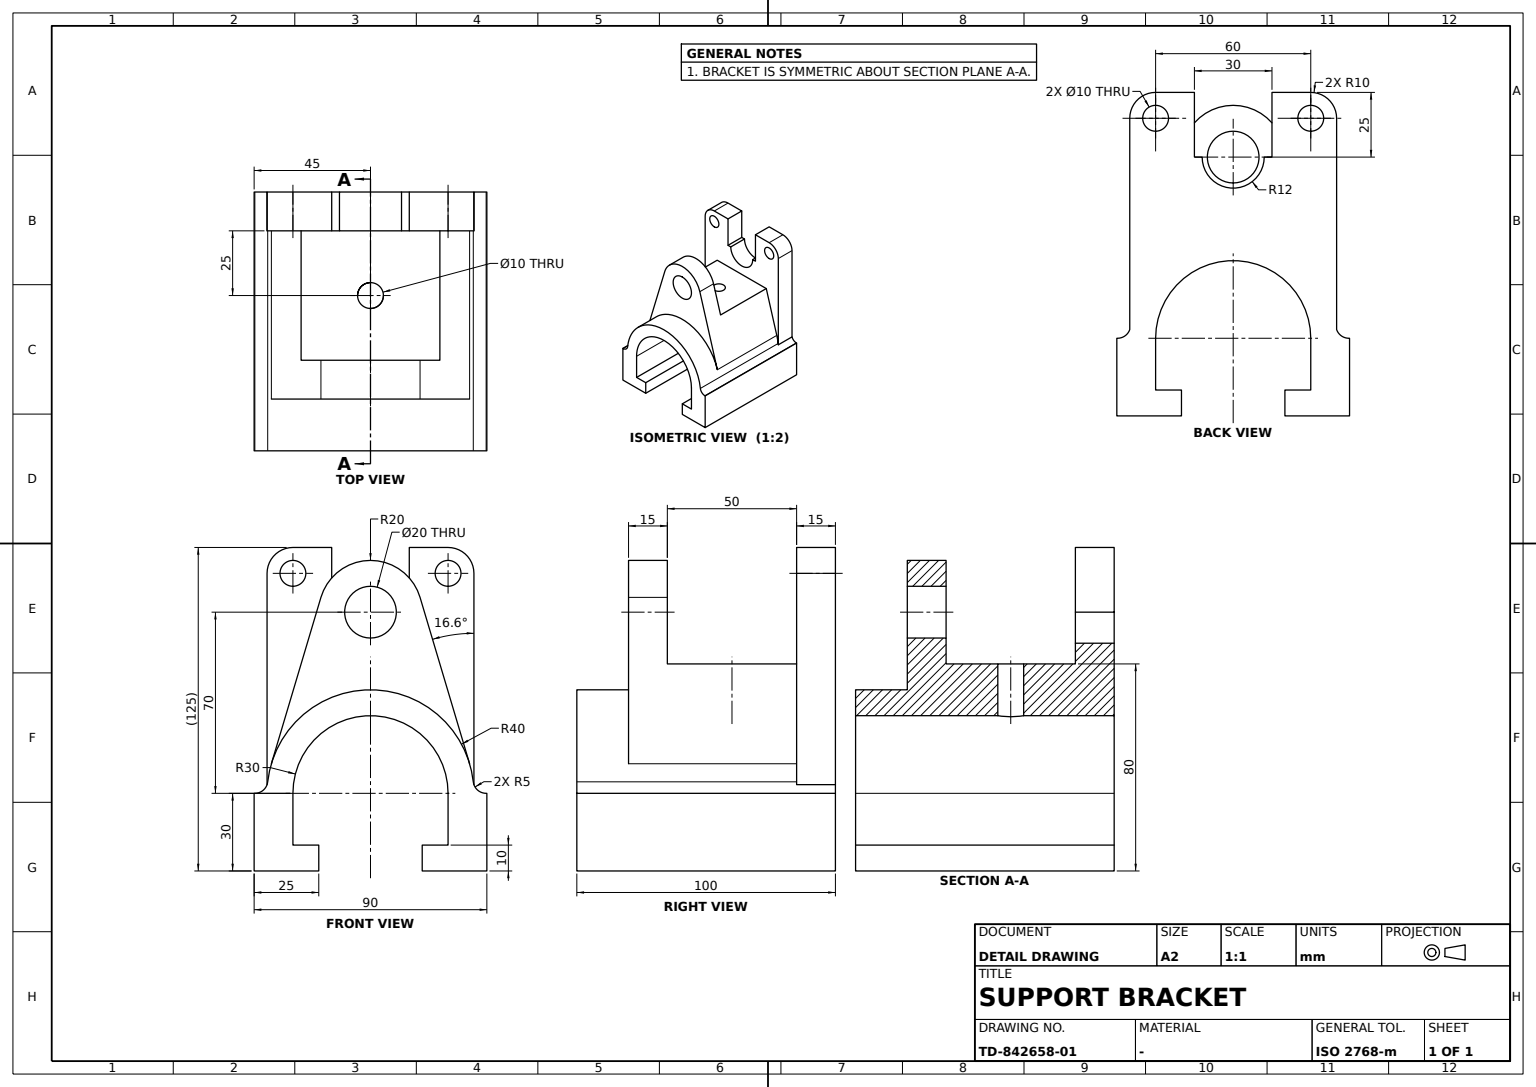
ISO-10303-21;
HEADER;
FILE_DESCRIPTION((''),'2;1');
FILE_NAME('','',(''),(''),'','','');
FILE_SCHEMA(('AUTOMOTIVE_DESIGN'));
ENDSEC;
DATA;
#1=APPLICATION_CONTEXT('');
#2=PRODUCT_CONTEXT('',#1,'mechanical');
#3=PRODUCT('','','',(#2));
#4=PRODUCT_DEFINITION_FORMATION('','',#3);
#5=PRODUCT_DEFINITION_CONTEXT('',#1,'design');
#6=PRODUCT_DEFINITION('','',#4,#5);
#7=PRODUCT_DEFINITION_SHAPE('','',#6);
#8=(LENGTH_UNIT()NAMED_UNIT(*)SI_UNIT(.MILLI.,.METRE.));
#9=(NAMED_UNIT(*)PLANE_ANGLE_UNIT()SI_UNIT($,.RADIAN.));
#10=(NAMED_UNIT(*)SI_UNIT($,.STERADIAN.)SOLID_ANGLE_UNIT());
#11=UNCERTAINTY_MEASURE_WITH_UNIT(LENGTH_MEASURE(0.005),#8,'distance_accuracy_value','');
#12=(GEOMETRIC_REPRESENTATION_CONTEXT(3)GLOBAL_UNCERTAINTY_ASSIGNED_CONTEXT((#11))GLOBAL_UNIT_ASSIGNED_CONTEXT((#8,#9,#10))REPRESENTATION_CONTEXT('',''));
#13=CARTESIAN_POINT('',(38.332594,-35.,41.428571));
#14=VERTEX_POINT('',#13);
#15=CARTESIAN_POINT('',(38.332594,30.,41.428571));
#16=VERTEX_POINT('',#15);
#17=CARTESIAN_POINT('',(38.332594,0.,41.428571));
#18=DIRECTION('',(0.,1.,0.));
#19=VECTOR('',#18,1000.);
#20=LINE('',#17,#19);
#21=EDGE_CURVE('',#14,#16,#20,.T.);
#22=ORIENTED_EDGE('',*,*,#21,.F.);
#23=CARTESIAN_POINT('',(39.75232,-35.,34.444444));
#24=VERTEX_POINT('',#23);
#25=CARTESIAN_POINT('',(0.,-35.,30.));
#26=DIRECTION('',(0.,-1.,0.));
#27=DIRECTION('',(0.,0.,-1.));
#28=AXIS2_PLACEMENT_3D('',#25,#26,#27);
#29=CIRCLE('',#28,40.);
#30=EDGE_CURVE('',#24,#14,#29,.T.);
#31=ORIENTED_EDGE('',*,*,#30,.F.);
#32=CARTESIAN_POINT('',(39.75232,50.,34.444444));
#33=VERTEX_POINT('',#32);
#34=CARTESIAN_POINT('',(39.75232,7.5,34.444444));
#35=LINE('',#34,#19);
#36=EDGE_CURVE('',#24,#33,#35,.T.);
#37=ORIENTED_EDGE('',*,*,#36,.T.);
#38=CARTESIAN_POINT('',(-39.75232,50.,34.444444));
#39=VERTEX_POINT('',#38);
#40=CARTESIAN_POINT('',(0.,50.,30.));
#41=DIRECTION('',(0.,0.,1.));
#42=AXIS2_PLACEMENT_3D('',#40,#18,#41);
#43=CIRCLE('',#42,40.);
#44=EDGE_CURVE('',#39,#33,#43,.T.);
#45=ORIENTED_EDGE('',*,*,#44,.F.);
#46=CARTESIAN_POINT('',(-39.75232,-35.,34.444444));
#47=VERTEX_POINT('',#46);
#48=CARTESIAN_POINT('',(-39.75232,7.5,34.444444));
#49=LINE('',#48,#19);
#50=EDGE_CURVE('',#47,#39,#49,.T.);
#51=ORIENTED_EDGE('',*,*,#50,.F.);
#52=CARTESIAN_POINT('',(-38.332594,-35.,41.428571));
#53=VERTEX_POINT('',#52);
#54=EDGE_CURVE('',#53,#47,#29,.T.);
#55=ORIENTED_EDGE('',*,*,#54,.F.);
#56=CARTESIAN_POINT('',(-38.332594,30.,41.428571));
#57=VERTEX_POINT('',#56);
#58=CARTESIAN_POINT('',(-38.332594,0.,41.428571));
#59=LINE('',#58,#19);
#60=EDGE_CURVE('',#53,#57,#59,.T.);
#61=ORIENTED_EDGE('',*,*,#60,.T.);
#62=CARTESIAN_POINT('',(0.,30.,30.));
#63=AXIS2_PLACEMENT_3D('',#62,#18,#41);
#64=CIRCLE('',#63,40.);
#65=EDGE_CURVE('',#57,#16,#64,.T.);
#66=ORIENTED_EDGE('',*,*,#65,.T.);
#67=EDGE_LOOP('',(#22,#31,#37,#45,#51,#55,#61,#66));
#68=FACE_BOUND('',#67,.T.);
#69=CARTESIAN_POINT('',(0.,0.,30.));
#70=DIRECTION('',(-1.,0.,0.));
#71=AXIS2_PLACEMENT_3D('',#69,#18,#70);
#72=CYLINDRICAL_SURFACE('',#71,40.);
#73=ADVANCED_FACE('',(#68),#72,.T.);
#74=CARTESIAN_POINT('',(44.72136,50.,30.));
#75=VERTEX_POINT('',#74);
#76=CARTESIAN_POINT('',(45.,50.,30.));
#77=VERTEX_POINT('',#76);
#78=DIRECTION('',(1.,0.,0.));
#79=VECTOR('',#78,1000.);
#80=LINE('',#40,#79);
#81=EDGE_CURVE('',#75,#77,#80,.T.);
#82=ORIENTED_EDGE('',*,*,#81,.T.);
#83=CARTESIAN_POINT('',(45.,50.,0.));
#84=VERTEX_POINT('',#83);
#85=VECTOR('',#27,1000.);
#86=LINE('',#83,#85);
#87=EDGE_CURVE('',#77,#84,#86,.T.);
#88=ORIENTED_EDGE('',*,*,#87,.T.);
#89=CARTESIAN_POINT('',(20.,50.,0.));
#90=VERTEX_POINT('',#89);
#91=CARTESIAN_POINT('',(0.,50.,0.));
#92=VECTOR('',#70,1000.);
#93=LINE('',#91,#92);
#94=EDGE_CURVE('',#84,#90,#93,.T.);
#95=ORIENTED_EDGE('',*,*,#94,.T.);
#96=CARTESIAN_POINT('',(20.,50.,10.));
#97=VERTEX_POINT('',#96);
#98=VECTOR('',#41,1000.);
#99=LINE('',#89,#98);
#100=EDGE_CURVE('',#90,#97,#99,.T.);
#101=ORIENTED_EDGE('',*,*,#100,.T.);
#102=CARTESIAN_POINT('',(30.,50.,10.));
#103=VERTEX_POINT('',#102);
#104=CARTESIAN_POINT('',(0.,50.,10.));
#105=LINE('',#104,#79);
#106=EDGE_CURVE('',#97,#103,#105,.T.);
#107=ORIENTED_EDGE('',*,*,#106,.T.);
#108=CARTESIAN_POINT('',(30.,50.,30.));
#109=VERTEX_POINT('',#108);
#110=CARTESIAN_POINT('',(30.,50.,0.));
#111=LINE('',#110,#98);
#112=EDGE_CURVE('',#103,#109,#111,.T.);
#113=ORIENTED_EDGE('',*,*,#112,.T.);
#114=CARTESIAN_POINT('',(-30.,50.,30.));
#115=VERTEX_POINT('',#114);
#116=CIRCLE('',#42,30.);
#117=EDGE_CURVE('',#115,#109,#116,.T.);
#118=ORIENTED_EDGE('',*,*,#117,.F.);
#119=CARTESIAN_POINT('',(-30.,50.,10.));
#120=VERTEX_POINT('',#119);
#121=CARTESIAN_POINT('',(-30.,50.,0.));
#122=LINE('',#121,#98);
#123=EDGE_CURVE('',#120,#115,#122,.T.);
#124=ORIENTED_EDGE('',*,*,#123,.F.);
#125=CARTESIAN_POINT('',(-20.,50.,10.));
#126=VERTEX_POINT('',#125);
#127=LINE('',#96,#92);
#128=EDGE_CURVE('',#126,#120,#127,.T.);
#129=ORIENTED_EDGE('',*,*,#128,.F.);
#130=CARTESIAN_POINT('',(-20.,50.,0.));
#131=VERTEX_POINT('',#130);
#132=LINE('',#130,#98);
#133=EDGE_CURVE('',#131,#126,#132,.T.);
#134=ORIENTED_EDGE('',*,*,#133,.F.);
#135=CARTESIAN_POINT('',(-45.,50.,0.));
#136=VERTEX_POINT('',#135);
#137=EDGE_CURVE('',#131,#136,#93,.T.);
#138=ORIENTED_EDGE('',*,*,#137,.T.);
#139=CARTESIAN_POINT('',(-45.,50.,30.));
#140=VERTEX_POINT('',#139);
#141=LINE('',#135,#98);
#142=EDGE_CURVE('',#136,#140,#141,.T.);
#143=ORIENTED_EDGE('',*,*,#142,.T.);
#144=CARTESIAN_POINT('',(-44.72136,50.,30.));
#145=VERTEX_POINT('',#144);
#146=EDGE_CURVE('',#140,#145,#80,.T.);
#147=ORIENTED_EDGE('',*,*,#146,.T.);
#148=CARTESIAN_POINT('',(-44.72136,50.,35.));
#149=AXIS2_PLACEMENT_3D('',#148,#18,#41);
#150=CIRCLE('',#149,5.);
#151=EDGE_CURVE('',#39,#145,#150,.T.);
#152=ORIENTED_EDGE('',*,*,#151,.F.);
#153=ORIENTED_EDGE('',*,*,#44,.T.);
#154=CARTESIAN_POINT('',(44.72136,50.,35.));
#155=AXIS2_PLACEMENT_3D('',#154,#18,#41);
#156=CIRCLE('',#155,5.);
#157=EDGE_CURVE('',#75,#33,#156,.T.);
#158=ORIENTED_EDGE('',*,*,#157,.F.);
#159=EDGE_LOOP('',(#82,#88,#95,#101,#107,#113,#118,#124,#129,#134,#138,#143,#147,#152,#153,#158));
#160=FACE_BOUND('',#159,.T.);
#161=AXIS2_PLACEMENT_3D('',#91,#18,#70);
#162=PLANE('',#161);
#163=ADVANCED_FACE('',(#160),#162,.T.);
#164=CARTESIAN_POINT('',(40.,-35.,33.354168));
#165=VERTEX_POINT('',#164);
#166=CARTESIAN_POINT('',(40.,-35.,115.));
#167=VERTEX_POINT('',#166);
#168=CARTESIAN_POINT('',(40.,-35.,30.));
#169=LINE('',#168,#98);
#170=EDGE_CURVE('',#165,#167,#169,.T.);
#171=ORIENTED_EDGE('',*,*,#170,.T.);
#172=CARTESIAN_POINT('',(40.,-50.,115.));
#173=VERTEX_POINT('',#172);
#174=CARTESIAN_POINT('',(40.,-42.5,115.));
#175=VECTOR('',#26,1000.);
#176=LINE('',#174,#175);
#177=EDGE_CURVE('',#173,#167,#176,.F.);
#178=ORIENTED_EDGE('',*,*,#177,.F.);
#179=CARTESIAN_POINT('',(40.,-50.,33.354168));
#180=VERTEX_POINT('',#179);
#181=CARTESIAN_POINT('',(40.,-50.,0.));
#182=LINE('',#181,#98);
#183=EDGE_CURVE('',#180,#173,#182,.T.);
#184=ORIENTED_EDGE('',*,*,#183,.F.);
#185=LINE('',#164,#19);
#186=EDGE_CURVE('',#165,#180,#185,.F.);
#187=ORIENTED_EDGE('',*,*,#186,.F.);
#188=EDGE_LOOP('',(#171,#178,#184,#187));
#189=FACE_BOUND('',#188,.T.);
#190=CARTESIAN_POINT('',(40.,-50.,30.));
#191=AXIS2_PLACEMENT_3D('',#190,#70,#41);
#192=PLANE('',#191);
#193=ADVANCED_FACE('',(#189),#192,.F.);
#194=CARTESIAN_POINT('',(-26.832816,15.,80.));
#195=VERTEX_POINT('',#194);
#196=CARTESIAN_POINT('',(-19.166297,15.,105.714286));
#197=VERTEX_POINT('',#196);
#198=CARTESIAN_POINT('',(-38.332594,15.,41.428571));
#199=DIRECTION('',(0.285714286,0.,0.958314847));
#200=VECTOR('',#199,1000.);
#201=LINE('',#198,#200);
#202=EDGE_CURVE('',#195,#197,#201,.T.);
#203=ORIENTED_EDGE('',*,*,#202,.F.);
#204=CARTESIAN_POINT('',(26.832816,15.,80.));
#205=VERTEX_POINT('',#204);
#206=CARTESIAN_POINT('',(0.,15.,80.));
#207=LINE('',#206,#92);
#208=EDGE_CURVE('',#205,#195,#207,.T.);
#209=ORIENTED_EDGE('',*,*,#208,.F.);
#210=CARTESIAN_POINT('',(19.166297,15.,105.714286));
#211=VERTEX_POINT('',#210);
#212=CARTESIAN_POINT('',(46.546721,15.,13.877551));
#213=DIRECTION('',(0.285714286,0.,-0.958314847));
#214=VECTOR('',#213,1000.);
#215=LINE('',#212,#214);
#216=EDGE_CURVE('',#211,#205,#215,.T.);
#217=ORIENTED_EDGE('',*,*,#216,.F.);
#218=CARTESIAN_POINT('',(0.,15.,100.));
#219=AXIS2_PLACEMENT_3D('',#218,#26,#27);
#220=CIRCLE('',#219,20.);
#221=EDGE_CURVE('',#211,#197,#220,.T.);
#222=ORIENTED_EDGE('',*,*,#221,.T.);
#223=EDGE_LOOP('',(#203,#209,#217,#222));
#224=FACE_BOUND('',#223,.T.);
#225=CARTESIAN_POINT('',(0.,15.,90.));
#226=VERTEX_POINT('',#225);
#227=CIRCLE('',#219,10.);
#228=EDGE_CURVE('',#226,#226,#227,.T.);
#229=ORIENTED_EDGE('',*,*,#228,.F.);
#230=EDGE_LOOP('',(#229));
#231=FACE_BOUND('',#230,.T.);
#232=CARTESIAN_POINT('',(0.,15.,0.));
#233=AXIS2_PLACEMENT_3D('',#232,#26,#78);
#234=PLANE('',#233);
#235=ADVANCED_FACE('',(#224,#231),#234,.T.);
#236=CARTESIAN_POINT('',(-19.166297,30.,105.714286));
#237=VERTEX_POINT('',#236);
#238=CARTESIAN_POINT('',(19.166297,30.,105.714286));
#239=VERTEX_POINT('',#238);
#240=CARTESIAN_POINT('',(0.,30.,100.));
#241=AXIS2_PLACEMENT_3D('',#240,#18,#41);
#242=CIRCLE('',#241,20.);
#243=EDGE_CURVE('',#237,#239,#242,.T.);
#244=ORIENTED_EDGE('',*,*,#243,.F.);
#245=LINE('',#196,#19);
#246=EDGE_CURVE('',#197,#237,#245,.T.);
#247=ORIENTED_EDGE('',*,*,#246,.F.);
#248=ORIENTED_EDGE('',*,*,#221,.F.);
#249=LINE('',#210,#19);
#250=EDGE_CURVE('',#211,#239,#249,.T.);
#251=ORIENTED_EDGE('',*,*,#250,.T.);
#252=EDGE_LOOP('',(#244,#247,#248,#251));
#253=FACE_BOUND('',#252,.T.);
#254=AXIS2_PLACEMENT_3D('',#218,#18,#70);
#255=CYLINDRICAL_SURFACE('',#254,20.);
#256=ADVANCED_FACE('',(#253),#255,.T.);
#257=CARTESIAN_POINT('',(20.,-50.,10.));
#258=VERTEX_POINT('',#257);
#259=CARTESIAN_POINT('',(20.,0.,10.));
#260=LINE('',#259,#19);
#261=EDGE_CURVE('',#258,#97,#260,.T.);
#262=ORIENTED_EDGE('',*,*,#261,.F.);
#263=CARTESIAN_POINT('',(30.,-50.,10.));
#264=VERTEX_POINT('',#263);
#265=CARTESIAN_POINT('',(0.,-50.,10.));
#266=LINE('',#265,#79);
#267=EDGE_CURVE('',#258,#264,#266,.T.);
#268=ORIENTED_EDGE('',*,*,#267,.T.);
#269=CARTESIAN_POINT('',(30.,0.,10.));
#270=LINE('',#269,#19);
#271=EDGE_CURVE('',#264,#103,#270,.T.);
#272=ORIENTED_EDGE('',*,*,#271,.T.);
#273=ORIENTED_EDGE('',*,*,#106,.F.);
#274=EDGE_LOOP('',(#262,#268,#272,#273));
#275=FACE_BOUND('',#274,.T.);
#276=AXIS2_PLACEMENT_3D('',#259,#41,#78);
#277=PLANE('',#276);
#278=ADVANCED_FACE('',(#275),#277,.T.);
#279=CARTESIAN_POINT('',(5.,-10.,80.));
#280=VERTEX_POINT('',#279);
#281=CARTESIAN_POINT('',(0.,-10.,80.));
#282=AXIS2_PLACEMENT_3D('',#281,#41,#78);
#283=CIRCLE('',#282,5.);
#284=EDGE_CURVE('',#280,#280,#283,.T.);
#285=ORIENTED_EDGE('',*,*,#284,.T.);
#286=EDGE_LOOP('',(#285));
#287=FACE_BOUND('',#286,.T.);
#288=CARTESIAN_POINT('',(-5.,-10.,59.580399));
#289=VERTEX_POINT('',#288);
#290=CARTESIAN_POINT('',(-3.916178,-6.078413,59.792106));
#291=CARTESIAN_POINT('',(-5.541877,-10.000858,59.474634));
#292=CARTESIAN_POINT('',(-3.916314,-13.918153,59.79175));
#293=CARTESIAN_POINT('',(-0.005741,-15.540062,60.104036));
#294=CARTESIAN_POINT('',(3.916175,-13.921588,59.792107));
#295=CARTESIAN_POINT('',(5.541877,-9.999149,59.474634));
#296=CARTESIAN_POINT('',(3.916316,-6.081848,59.791749));
#297=CARTESIAN_POINT('',(0.005741,-4.459937,60.104036));
#298=B_SPLINE_CURVE_WITH_KNOTS('',3,(#290,#291,#292,#293,#294,#295,#296,#297,#290,#291,#292),.UNSPECIFIED.,.T.,.F.,(1,1,1,1,1,1,1,1,1,1,1,1,1,1,1),(-0.011741759,-0.007827839,-0.00391392,0.,0.00391392,0.007827839,0.011741759,0.015655678,0.019569598,0.023483517,0.027397437,0.031311356,0.035225276,0.039139195,0.043053115),.UNSPECIFIED.);
#299=EDGE_CURVE('',#289,#289,#298,.T.);
#300=ORIENTED_EDGE('',*,*,#299,.F.);
#301=EDGE_LOOP('',(#300));
#302=FACE_BOUND('',#301,.T.);
#303=CARTESIAN_POINT('',(0.,-10.,63.16));
#304=AXIS2_PLACEMENT_3D('',#303,#41,#78);
#305=CYLINDRICAL_SURFACE('',#304,5.);
#306=ADVANCED_FACE('',(#287,#302),#305,.F.);
#307=CARTESIAN_POINT('',(-40.,-50.,115.));
#308=VERTEX_POINT('',#307);
#309=CARTESIAN_POINT('',(-40.,-35.,115.));
#310=VERTEX_POINT('',#309);
#311=CARTESIAN_POINT('',(-40.,-42.5,115.));
#312=LINE('',#311,#175);
#313=EDGE_CURVE('',#308,#310,#312,.F.);
#314=ORIENTED_EDGE('',*,*,#313,.F.);
#315=CARTESIAN_POINT('',(-30.,-50.,125.));
#316=VERTEX_POINT('',#315);
#317=CARTESIAN_POINT('',(-30.,-50.,115.));
#318=AXIS2_PLACEMENT_3D('',#317,#18,#41);
#319=CIRCLE('',#318,10.);
#320=EDGE_CURVE('',#316,#308,#319,.F.);
#321=ORIENTED_EDGE('',*,*,#320,.F.);
#322=CARTESIAN_POINT('',(-30.,-35.,125.));
#323=VERTEX_POINT('',#322);
#324=CARTESIAN_POINT('',(-30.,-42.5,125.));
#325=LINE('',#324,#175);
#326=EDGE_CURVE('',#316,#323,#325,.F.);
#327=ORIENTED_EDGE('',*,*,#326,.T.);
#328=CARTESIAN_POINT('',(-30.,-35.,115.));
#329=AXIS2_PLACEMENT_3D('',#328,#26,#27);
#330=CIRCLE('',#329,10.);
#331=EDGE_CURVE('',#323,#310,#330,.T.);
#332=ORIENTED_EDGE('',*,*,#331,.T.);
#333=EDGE_LOOP('',(#314,#321,#327,#332));
#334=FACE_BOUND('',#333,.T.);
#335=CARTESIAN_POINT('',(-30.,-42.5,115.));
#336=AXIS2_PLACEMENT_3D('',#335,#26,#78);
#337=CYLINDRICAL_SURFACE('',#336,10.);
#338=ADVANCED_FACE('',(#334),#337,.T.);
#339=CARTESIAN_POINT('',(-20.,-50.,0.));
#340=VERTEX_POINT('',#339);
#341=CARTESIAN_POINT('',(-45.,-50.,0.));
#342=VERTEX_POINT('',#341);
#343=CARTESIAN_POINT('',(0.,-50.,0.));
#344=LINE('',#343,#92);
#345=EDGE_CURVE('',#340,#342,#344,.T.);
#346=ORIENTED_EDGE('',*,*,#345,.T.);
#347=CARTESIAN_POINT('',(-45.,0.,0.));
#348=LINE('',#347,#19);
#349=EDGE_CURVE('',#342,#136,#348,.T.);
#350=ORIENTED_EDGE('',*,*,#349,.T.);
#351=ORIENTED_EDGE('',*,*,#137,.F.);
#352=CARTESIAN_POINT('',(-20.,0.,0.));
#353=LINE('',#352,#19);
#354=EDGE_CURVE('',#340,#131,#353,.T.);
#355=ORIENTED_EDGE('',*,*,#354,.F.);
#356=EDGE_LOOP('',(#346,#350,#351,#355));
#357=FACE_BOUND('',#356,.T.);
#358=CARTESIAN_POINT('',(45.,0.,0.));
#359=AXIS2_PLACEMENT_3D('',#358,#27,#70);
#360=PLANE('',#359);
#361=ADVANCED_FACE('',(#357),#360,.T.);
#362=ORIENTED_EDGE('',*,*,#331,.F.);
#363=CARTESIAN_POINT('',(-15.,-35.,125.));
#364=VERTEX_POINT('',#363);
#365=CARTESIAN_POINT('',(30.,-35.,125.));
#366=LINE('',#365,#92);
#367=EDGE_CURVE('',#364,#323,#366,.T.);
#368=ORIENTED_EDGE('',*,*,#367,.F.);
#369=CARTESIAN_POINT('',(-15.,-35.,100.));
#370=VERTEX_POINT('',#369);
#371=LINE('',#363,#85);
#372=EDGE_CURVE('',#364,#370,#371,.T.);
#373=ORIENTED_EDGE('',*,*,#372,.T.);
#374=CARTESIAN_POINT('',(-12.,-35.,100.));
#375=VERTEX_POINT('',#374);
#376=CARTESIAN_POINT('',(12.,-35.,100.));
#377=LINE('',#376,#79);
#378=EDGE_CURVE('',#370,#375,#377,.T.);
#379=ORIENTED_EDGE('',*,*,#378,.T.);
#380=VERTEX_POINT('',#376);
#381=CARTESIAN_POINT('',(0.,-35.,100.));
#382=AXIS2_PLACEMENT_3D('',#381,#26,#27);
#383=CIRCLE('',#382,12.);
#384=EDGE_CURVE('',#375,#380,#383,.T.);
#385=ORIENTED_EDGE('',*,*,#384,.T.);
#386=CARTESIAN_POINT('',(15.,-35.,100.));
#387=VERTEX_POINT('',#386);
#388=EDGE_CURVE('',#380,#387,#377,.T.);
#389=ORIENTED_EDGE('',*,*,#388,.T.);
#390=CARTESIAN_POINT('',(15.,-35.,125.));
#391=VERTEX_POINT('',#390);
#392=LINE('',#386,#98);
#393=EDGE_CURVE('',#387,#391,#392,.T.);
#394=ORIENTED_EDGE('',*,*,#393,.T.);
#395=VERTEX_POINT('',#365);
#396=EDGE_CURVE('',#395,#391,#366,.T.);
#397=ORIENTED_EDGE('',*,*,#396,.F.);
#398=CARTESIAN_POINT('',(30.,-35.,115.));
#399=AXIS2_PLACEMENT_3D('',#398,#26,#27);
#400=CIRCLE('',#399,10.);
#401=EDGE_CURVE('',#167,#395,#400,.T.);
#402=ORIENTED_EDGE('',*,*,#401,.F.);
#403=ORIENTED_EDGE('',*,*,#170,.F.);
#404=CARTESIAN_POINT('',(44.72136,-35.,35.));
#405=AXIS2_PLACEMENT_3D('',#404,#26,#27);
#406=CIRCLE('',#405,5.);
#407=EDGE_CURVE('',#24,#165,#406,.T.);
#408=ORIENTED_EDGE('',*,*,#407,.F.);
#409=ORIENTED_EDGE('',*,*,#30,.T.);
#410=CARTESIAN_POINT('',(26.832816,-35.,80.));
#411=VERTEX_POINT('',#410);
#412=DIRECTION('',(-0.285714286,0.,0.958314847));
#413=VECTOR('',#412,1000.);
#414=LINE('',#13,#413);
#415=EDGE_CURVE('',#14,#411,#414,.T.);
#416=ORIENTED_EDGE('',*,*,#415,.T.);
#417=CARTESIAN_POINT('',(-26.832816,-35.,80.));
#418=VERTEX_POINT('',#417);
#419=CARTESIAN_POINT('',(0.,-35.,80.));
#420=LINE('',#419,#92);
#421=EDGE_CURVE('',#411,#418,#420,.T.);
#422=ORIENTED_EDGE('',*,*,#421,.T.);
#423=LINE('',#52,#200);
#424=EDGE_CURVE('',#53,#418,#423,.T.);
#425=ORIENTED_EDGE('',*,*,#424,.F.);
#426=ORIENTED_EDGE('',*,*,#54,.T.);
#427=CARTESIAN_POINT('',(-40.,-35.,33.354168));
#428=VERTEX_POINT('',#427);
#429=CARTESIAN_POINT('',(-44.72136,-35.,35.));
#430=AXIS2_PLACEMENT_3D('',#429,#26,#27);
#431=CIRCLE('',#430,5.);
#432=EDGE_CURVE('',#428,#47,#431,.T.);
#433=ORIENTED_EDGE('',*,*,#432,.F.);
#434=LINE('',#309,#85);
#435=EDGE_CURVE('',#310,#428,#434,.T.);
#436=ORIENTED_EDGE('',*,*,#435,.F.);
#437=EDGE_LOOP('',(#362,#368,#373,#379,#385,#389,#394,#397,#402,#403,#408,#409,#416,#422,#425,#426,#433,#436));
#438=FACE_BOUND('',#437,.T.);
#439=CARTESIAN_POINT('',(-30.,-35.,110.));
#440=VERTEX_POINT('',#439);
#441=CIRCLE('',#329,5.);
#442=EDGE_CURVE('',#440,#440,#441,.T.);
#443=ORIENTED_EDGE('',*,*,#442,.T.);
#444=EDGE_LOOP('',(#443));
#445=FACE_BOUND('',#444,.T.);
#446=CARTESIAN_POINT('',(30.,-35.,110.));
#447=VERTEX_POINT('',#446);
#448=CIRCLE('',#399,5.);
#449=EDGE_CURVE('',#447,#447,#448,.T.);
#450=ORIENTED_EDGE('',*,*,#449,.T.);
#451=EDGE_LOOP('',(#450));
#452=FACE_BOUND('',#451,.T.);
#453=CARTESIAN_POINT('',(0.,-35.,0.));
#454=AXIS2_PLACEMENT_3D('',#453,#26,#78);
#455=PLANE('',#454);
#456=ADVANCED_FACE('',(#438,#445,#452),#455,.F.);
#457=CARTESIAN_POINT('',(-15.,-50.,125.));
#458=VERTEX_POINT('',#457);
#459=LINE('',#457,#19);
#460=EDGE_CURVE('',#458,#364,#459,.T.);
#461=ORIENTED_EDGE('',*,*,#460,.F.);
#462=CARTESIAN_POINT('',(-15.,-50.,100.));
#463=VERTEX_POINT('',#462);
#464=CARTESIAN_POINT('',(-15.,-50.,0.));
#465=LINE('',#464,#85);
#466=EDGE_CURVE('',#458,#463,#465,.T.);
#467=ORIENTED_EDGE('',*,*,#466,.T.);
#468=LINE('',#462,#19);
#469=EDGE_CURVE('',#463,#370,#468,.T.);
#470=ORIENTED_EDGE('',*,*,#469,.T.);
#471=ORIENTED_EDGE('',*,*,#372,.F.);
#472=EDGE_LOOP('',(#461,#467,#470,#471));
#473=FACE_BOUND('',#472,.T.);
#474=AXIS2_PLACEMENT_3D('',#457,#78,#27);
#475=PLANE('',#474);
#476=ADVANCED_FACE('',(#473),#475,.T.);
#477=CARTESIAN_POINT('',(0.,30.,110.));
#478=VERTEX_POINT('',#477);
#479=CIRCLE('',#241,10.);
#480=EDGE_CURVE('',#478,#478,#479,.T.);
#481=ORIENTED_EDGE('',*,*,#480,.T.);
#482=EDGE_LOOP('',(#481));
#483=FACE_BOUND('',#482,.T.);
#484=ORIENTED_EDGE('',*,*,#228,.T.);
#485=EDGE_LOOP('',(#484));
#486=FACE_BOUND('',#485,.T.);
#487=CYLINDRICAL_SURFACE('',#254,10.);
#488=ADVANCED_FACE('',(#483,#486),#487,.F.);
#489=ORIENTED_EDGE('',*,*,#284,.F.);
#490=EDGE_LOOP('',(#489));
#491=FACE_BOUND('',#490,.T.);
#492=ORIENTED_EDGE('',*,*,#421,.F.);
#493=CARTESIAN_POINT('',(26.832816,0.,80.));
#494=LINE('',#493,#175);
#495=EDGE_CURVE('',#205,#411,#494,.T.);
#496=ORIENTED_EDGE('',*,*,#495,.F.);
#497=ORIENTED_EDGE('',*,*,#208,.T.);
#498=CARTESIAN_POINT('',(-26.832816,0.,80.));
#499=LINE('',#498,#175);
#500=EDGE_CURVE('',#195,#418,#499,.T.);
#501=ORIENTED_EDGE('',*,*,#500,.T.);
#502=EDGE_LOOP('',(#492,#496,#497,#501));
#503=FACE_BOUND('',#502,.T.);
#504=AXIS2_PLACEMENT_3D('',#493,#41,#70);
#505=PLANE('',#504);
#506=ADVANCED_FACE('',(#491,#503),#505,.T.);
#507=CARTESIAN_POINT('',(-30.,-50.,120.));
#508=VERTEX_POINT('',#507);
#509=CIRCLE('',#318,5.);
#510=EDGE_CURVE('',#508,#508,#509,.F.);
#511=ORIENTED_EDGE('',*,*,#510,.F.);
#512=EDGE_LOOP('',(#511));
#513=FACE_BOUND('',#512,.T.);
#514=CARTESIAN_POINT('',(30.,-50.,125.));
#515=VERTEX_POINT('',#514);
#516=CARTESIAN_POINT('',(30.,-50.,115.));
#517=AXIS2_PLACEMENT_3D('',#516,#18,#41);
#518=CIRCLE('',#517,10.);
#519=EDGE_CURVE('',#173,#515,#518,.F.);
#520=ORIENTED_EDGE('',*,*,#519,.T.);
#521=CARTESIAN_POINT('',(15.,-50.,125.));
#522=VERTEX_POINT('',#521);
#523=CARTESIAN_POINT('',(0.,-50.,125.));
#524=LINE('',#523,#92);
#525=EDGE_CURVE('',#515,#522,#524,.T.);
#526=ORIENTED_EDGE('',*,*,#525,.T.);
#527=CARTESIAN_POINT('',(15.,-50.,100.));
#528=VERTEX_POINT('',#527);
#529=CARTESIAN_POINT('',(15.,-50.,0.));
#530=LINE('',#529,#98);
#531=EDGE_CURVE('',#528,#522,#530,.T.);
#532=ORIENTED_EDGE('',*,*,#531,.F.);
#533=CARTESIAN_POINT('',(12.,-50.,100.));
#534=VERTEX_POINT('',#533);
#535=CARTESIAN_POINT('',(0.,-50.,100.));
#536=LINE('',#535,#79);
#537=EDGE_CURVE('',#534,#528,#536,.T.);
#538=ORIENTED_EDGE('',*,*,#537,.F.);
#539=CARTESIAN_POINT('',(-12.,-50.,100.));
#540=VERTEX_POINT('',#539);
#541=AXIS2_PLACEMENT_3D('',#535,#18,#41);
#542=CIRCLE('',#541,12.);
#543=EDGE_CURVE('',#540,#534,#542,.F.);
#544=ORIENTED_EDGE('',*,*,#543,.F.);
#545=EDGE_CURVE('',#463,#540,#536,.T.);
#546=ORIENTED_EDGE('',*,*,#545,.F.);
#547=ORIENTED_EDGE('',*,*,#466,.F.);
#548=EDGE_CURVE('',#458,#316,#524,.T.);
#549=ORIENTED_EDGE('',*,*,#548,.T.);
#550=ORIENTED_EDGE('',*,*,#320,.T.);
#551=CARTESIAN_POINT('',(-40.,-50.,33.354168));
#552=VERTEX_POINT('',#551);
#553=CARTESIAN_POINT('',(-40.,-50.,0.));
#554=LINE('',#553,#85);
#555=EDGE_CURVE('',#308,#552,#554,.T.);
#556=ORIENTED_EDGE('',*,*,#555,.T.);
#557=CARTESIAN_POINT('',(-44.72136,-50.,30.));
#558=VERTEX_POINT('',#557);
#559=CARTESIAN_POINT('',(-44.72136,-50.,35.));
#560=AXIS2_PLACEMENT_3D('',#559,#18,#41);
#561=CIRCLE('',#560,5.);
#562=EDGE_CURVE('',#552,#558,#561,.T.);
#563=ORIENTED_EDGE('',*,*,#562,.T.);
#564=CARTESIAN_POINT('',(-45.,-50.,30.));
#565=VERTEX_POINT('',#564);
#566=CARTESIAN_POINT('',(0.,-50.,30.));
#567=LINE('',#566,#79);
#568=EDGE_CURVE('',#565,#558,#567,.T.);
#569=ORIENTED_EDGE('',*,*,#568,.F.);
#570=LINE('',#341,#98);
#571=EDGE_CURVE('',#342,#565,#570,.T.);
#572=ORIENTED_EDGE('',*,*,#571,.F.);
#573=ORIENTED_EDGE('',*,*,#345,.F.);
#574=CARTESIAN_POINT('',(-20.,-50.,10.));
#575=VERTEX_POINT('',#574);
#576=LINE('',#339,#98);
#577=EDGE_CURVE('',#340,#575,#576,.T.);
#578=ORIENTED_EDGE('',*,*,#577,.T.);
#579=CARTESIAN_POINT('',(-30.,-50.,10.));
#580=VERTEX_POINT('',#579);
#581=LINE('',#257,#92);
#582=EDGE_CURVE('',#575,#580,#581,.T.);
#583=ORIENTED_EDGE('',*,*,#582,.T.);
#584=CARTESIAN_POINT('',(-30.,-50.,30.));
#585=VERTEX_POINT('',#584);
#586=CARTESIAN_POINT('',(-30.,-50.,0.));
#587=LINE('',#586,#98);
#588=EDGE_CURVE('',#580,#585,#587,.T.);
#589=ORIENTED_EDGE('',*,*,#588,.T.);
#590=CARTESIAN_POINT('',(30.,-50.,30.));
#591=VERTEX_POINT('',#590);
#592=AXIS2_PLACEMENT_3D('',#566,#18,#41);
#593=CIRCLE('',#592,30.);
#594=EDGE_CURVE('',#585,#591,#593,.T.);
#595=ORIENTED_EDGE('',*,*,#594,.T.);
#596=CARTESIAN_POINT('',(30.,-50.,0.));
#597=LINE('',#596,#98);
#598=EDGE_CURVE('',#264,#591,#597,.T.);
#599=ORIENTED_EDGE('',*,*,#598,.F.);
#600=ORIENTED_EDGE('',*,*,#267,.F.);
#601=CARTESIAN_POINT('',(20.,-50.,0.));
#602=VERTEX_POINT('',#601);
#603=LINE('',#601,#98);
#604=EDGE_CURVE('',#602,#258,#603,.T.);
#605=ORIENTED_EDGE('',*,*,#604,.F.);
#606=CARTESIAN_POINT('',(45.,-50.,0.));
#607=VERTEX_POINT('',#606);
#608=EDGE_CURVE('',#607,#602,#344,.T.);
#609=ORIENTED_EDGE('',*,*,#608,.F.);
#610=CARTESIAN_POINT('',(45.,-50.,30.));
#611=VERTEX_POINT('',#610);
#612=LINE('',#606,#85);
#613=EDGE_CURVE('',#611,#607,#612,.T.);
#614=ORIENTED_EDGE('',*,*,#613,.F.);
#615=CARTESIAN_POINT('',(44.72136,-50.,30.));
#616=VERTEX_POINT('',#615);
#617=EDGE_CURVE('',#616,#611,#567,.T.);
#618=ORIENTED_EDGE('',*,*,#617,.F.);
#619=CARTESIAN_POINT('',(44.72136,-50.,35.));
#620=AXIS2_PLACEMENT_3D('',#619,#18,#41);
#621=CIRCLE('',#620,5.);
#622=EDGE_CURVE('',#616,#180,#621,.T.);
#623=ORIENTED_EDGE('',*,*,#622,.T.);
#624=ORIENTED_EDGE('',*,*,#183,.T.);
#625=EDGE_LOOP('',(#520,#526,#532,#538,#544,#546,#547,#549,#550,#556,#563,#569,#572,#573,#578,#583,#589,#595,#599,#600,#605,#609,#614,#618,#623,#624));
#626=FACE_BOUND('',#625,.T.);
#627=CARTESIAN_POINT('',(30.,-50.,120.));
#628=VERTEX_POINT('',#627);
#629=CIRCLE('',#517,5.);
#630=EDGE_CURVE('',#628,#628,#629,.F.);
#631=ORIENTED_EDGE('',*,*,#630,.F.);
#632=EDGE_LOOP('',(#631));
#633=FACE_BOUND('',#632,.T.);
#634=AXIS2_PLACEMENT_3D('',#343,#18,#70);
#635=PLANE('',#634);
#636=ADVANCED_FACE('',(#513,#626,#633),#635,.F.);
#637=CARTESIAN_POINT('',(-20.,0.,10.));
#638=LINE('',#637,#19);
#639=EDGE_CURVE('',#575,#126,#638,.T.);
#640=ORIENTED_EDGE('',*,*,#639,.F.);
#641=ORIENTED_EDGE('',*,*,#577,.F.);
#642=ORIENTED_EDGE('',*,*,#354,.T.);
#643=ORIENTED_EDGE('',*,*,#133,.T.);
#644=EDGE_LOOP('',(#640,#641,#642,#643));
#645=FACE_BOUND('',#644,.T.);
#646=AXIS2_PLACEMENT_3D('',#352,#70,#41);
#647=PLANE('',#646);
#648=ADVANCED_FACE('',(#645),#647,.F.);
#649=ORIENTED_EDGE('',*,*,#571,.T.);
#650=CARTESIAN_POINT('',(-45.,0.,30.));
#651=LINE('',#650,#19);
#652=EDGE_CURVE('',#565,#140,#651,.T.);
#653=ORIENTED_EDGE('',*,*,#652,.T.);
#654=ORIENTED_EDGE('',*,*,#142,.F.);
#655=ORIENTED_EDGE('',*,*,#349,.F.);
#656=EDGE_LOOP('',(#649,#653,#654,#655));
#657=FACE_BOUND('',#656,.T.);
#658=AXIS2_PLACEMENT_3D('',#347,#70,#41);
#659=PLANE('',#658);
#660=ADVANCED_FACE('',(#657),#659,.T.);
#661=ORIENTED_EDGE('',*,*,#250,.F.);
#662=ORIENTED_EDGE('',*,*,#216,.T.);
#663=ORIENTED_EDGE('',*,*,#495,.T.);
#664=ORIENTED_EDGE('',*,*,#415,.F.);
#665=ORIENTED_EDGE('',*,*,#21,.T.);
#666=CARTESIAN_POINT('',(46.546721,30.,13.877551));
#667=LINE('',#666,#413);
#668=EDGE_CURVE('',#16,#239,#667,.T.);
#669=ORIENTED_EDGE('',*,*,#668,.T.);
#670=EDGE_LOOP('',(#661,#662,#663,#664,#665,#669));
#671=FACE_BOUND('',#670,.T.);
#672=DIRECTION('',(-0.958314847,0.,-0.285714286));
#673=AXIS2_PLACEMENT_3D('',#17,#672,#412);
#674=PLANE('',#673);
#675=ADVANCED_FACE('',(#671),#674,.F.);
#676=ORIENTED_EDGE('',*,*,#246,.T.);
#677=CARTESIAN_POINT('',(-46.546721,30.,13.877551));
#678=LINE('',#677,#200);
#679=EDGE_CURVE('',#57,#237,#678,.T.);
#680=ORIENTED_EDGE('',*,*,#679,.F.);
#681=ORIENTED_EDGE('',*,*,#60,.F.);
#682=ORIENTED_EDGE('',*,*,#424,.T.);
#683=ORIENTED_EDGE('',*,*,#500,.F.);
#684=ORIENTED_EDGE('',*,*,#202,.T.);
#685=EDGE_LOOP('',(#676,#680,#681,#682,#683,#684));
#686=FACE_BOUND('',#685,.T.);
#687=DIRECTION('',(-0.958314847,0.,0.285714286));
#688=AXIS2_PLACEMENT_3D('',#58,#687,#199);
#689=PLANE('',#688);
#690=ADVANCED_FACE('',(#686),#689,.T.);
#691=ORIENTED_EDGE('',*,*,#537,.T.);
#692=LINE('',#527,#19);
#693=EDGE_CURVE('',#528,#387,#692,.T.);
#694=ORIENTED_EDGE('',*,*,#693,.T.);
#695=ORIENTED_EDGE('',*,*,#388,.F.);
#696=LINE('',#533,#175);
#697=EDGE_CURVE('',#534,#380,#696,.F.);
#698=ORIENTED_EDGE('',*,*,#697,.F.);
#699=EDGE_LOOP('',(#691,#694,#695,#698));
#700=FACE_BOUND('',#699,.T.);
#701=AXIS2_PLACEMENT_3D('',#533,#41,#78);
#702=PLANE('',#701);
#703=ADVANCED_FACE('',(#700),#702,.T.);
#704=CARTESIAN_POINT('',(44.72136,0.,30.));
#705=LINE('',#704,#19);
#706=EDGE_CURVE('',#616,#75,#705,.T.);
#707=ORIENTED_EDGE('',*,*,#706,.F.);
#708=ORIENTED_EDGE('',*,*,#617,.T.);
#709=CARTESIAN_POINT('',(45.,0.,30.));
#710=LINE('',#709,#19);
#711=EDGE_CURVE('',#611,#77,#710,.T.);
#712=ORIENTED_EDGE('',*,*,#711,.T.);
#713=ORIENTED_EDGE('',*,*,#81,.F.);
#714=EDGE_LOOP('',(#707,#708,#712,#713));
#715=FACE_BOUND('',#714,.T.);
#716=AXIS2_PLACEMENT_3D('',#650,#41,#78);
#717=PLANE('',#716);
#718=ADVANCED_FACE('',(#715),#717,.T.);
#719=ORIENTED_EDGE('',*,*,#177,.T.);
#720=ORIENTED_EDGE('',*,*,#401,.T.);
#721=CARTESIAN_POINT('',(30.,-42.5,125.));
#722=LINE('',#721,#175);
#723=EDGE_CURVE('',#515,#395,#722,.F.);
#724=ORIENTED_EDGE('',*,*,#723,.F.);
#725=ORIENTED_EDGE('',*,*,#519,.F.);
#726=EDGE_LOOP('',(#719,#720,#724,#725));
#727=FACE_BOUND('',#726,.T.);
#728=CARTESIAN_POINT('',(30.,-42.5,115.));
#729=AXIS2_PLACEMENT_3D('',#728,#26,#78);
#730=CYLINDRICAL_SURFACE('',#729,10.);
#731=ADVANCED_FACE('',(#727),#730,.T.);
#732=ORIENTED_EDGE('',*,*,#510,.T.);
#733=EDGE_LOOP('',(#732));
#734=FACE_BOUND('',#733,.T.);
#735=ORIENTED_EDGE('',*,*,#442,.F.);
#736=EDGE_LOOP('',(#735));
#737=FACE_BOUND('',#736,.T.);
#738=CYLINDRICAL_SURFACE('',#336,5.);
#739=ADVANCED_FACE('',(#734,#737),#738,.F.);
#740=CARTESIAN_POINT('',(-44.72136,0.,30.));
#741=LINE('',#740,#19);
#742=EDGE_CURVE('',#558,#145,#741,.T.);
#743=ORIENTED_EDGE('',*,*,#742,.T.);
#744=ORIENTED_EDGE('',*,*,#146,.F.);
#745=ORIENTED_EDGE('',*,*,#652,.F.);
#746=ORIENTED_EDGE('',*,*,#568,.T.);
#747=EDGE_LOOP('',(#743,#744,#745,#746));
#748=FACE_BOUND('',#747,.T.);
#749=ADVANCED_FACE('',(#748),#717,.T.);
#750=ORIENTED_EDGE('',*,*,#326,.F.);
#751=ORIENTED_EDGE('',*,*,#548,.F.);
#752=ORIENTED_EDGE('',*,*,#460,.T.);
#753=ORIENTED_EDGE('',*,*,#367,.T.);
#754=EDGE_LOOP('',(#750,#751,#752,#753));
#755=FACE_BOUND('',#754,.T.);
#756=AXIS2_PLACEMENT_3D('',#514,#27,#70);
#757=PLANE('',#756);
#758=ADVANCED_FACE('',(#755),#757,.F.);
#759=ORIENTED_EDGE('',*,*,#432,.T.);
#760=ORIENTED_EDGE('',*,*,#50,.T.);
#761=ORIENTED_EDGE('',*,*,#151,.T.);
#762=ORIENTED_EDGE('',*,*,#742,.F.);
#763=ORIENTED_EDGE('',*,*,#562,.F.);
#764=LINE('',#427,#19);
#765=EDGE_CURVE('',#428,#552,#764,.F.);
#766=ORIENTED_EDGE('',*,*,#765,.F.);
#767=EDGE_LOOP('',(#759,#760,#761,#762,#763,#766));
#768=FACE_BOUND('',#767,.T.);
#769=CARTESIAN_POINT('',(-44.72136,0.,35.));
#770=DIRECTION('',(0.99380799,0.,-0.111111111));
#771=AXIS2_PLACEMENT_3D('',#769,#18,#770);
#772=CYLINDRICAL_SURFACE('',#771,5.);
#773=ADVANCED_FACE('',(#768),#772,.F.);
#774=ORIENTED_EDGE('',*,*,#588,.F.);
#775=CARTESIAN_POINT('',(-30.,0.,10.));
#776=LINE('',#775,#19);
#777=EDGE_CURVE('',#580,#120,#776,.T.);
#778=ORIENTED_EDGE('',*,*,#777,.T.);
#779=ORIENTED_EDGE('',*,*,#123,.T.);
#780=CARTESIAN_POINT('',(-30.,0.,30.));
#781=LINE('',#780,#19);
#782=EDGE_CURVE('',#585,#115,#781,.T.);
#783=ORIENTED_EDGE('',*,*,#782,.F.);
#784=EDGE_LOOP('',(#774,#778,#779,#783));
#785=FACE_BOUND('',#784,.T.);
#786=AXIS2_PLACEMENT_3D('',#775,#70,#41);
#787=PLANE('',#786);
#788=ADVANCED_FACE('',(#785),#787,.F.);
#789=ORIENTED_EDGE('',*,*,#613,.T.);
#790=LINE('',#358,#19);
#791=EDGE_CURVE('',#607,#84,#790,.T.);
#792=ORIENTED_EDGE('',*,*,#791,.T.);
#793=ORIENTED_EDGE('',*,*,#87,.F.);
#794=ORIENTED_EDGE('',*,*,#711,.F.);
#795=EDGE_LOOP('',(#789,#792,#793,#794));
#796=FACE_BOUND('',#795,.T.);
#797=AXIS2_PLACEMENT_3D('',#709,#78,#27);
#798=PLANE('',#797);
#799=ADVANCED_FACE('',(#796),#798,.T.);
#800=ORIENTED_EDGE('',*,*,#693,.F.);
#801=ORIENTED_EDGE('',*,*,#531,.T.);
#802=LINE('',#521,#19);
#803=EDGE_CURVE('',#522,#391,#802,.T.);
#804=ORIENTED_EDGE('',*,*,#803,.T.);
#805=ORIENTED_EDGE('',*,*,#393,.F.);
#806=EDGE_LOOP('',(#800,#801,#804,#805));
#807=FACE_BOUND('',#806,.T.);
#808=AXIS2_PLACEMENT_3D('',#527,#70,#41);
#809=PLANE('',#808);
#810=ADVANCED_FACE('',(#807),#809,.T.);
#811=ORIENTED_EDGE('',*,*,#469,.F.);
#812=ORIENTED_EDGE('',*,*,#545,.T.);
#813=LINE('',#539,#175);
#814=EDGE_CURVE('',#540,#375,#813,.F.);
#815=ORIENTED_EDGE('',*,*,#814,.T.);
#816=ORIENTED_EDGE('',*,*,#378,.F.);
#817=EDGE_LOOP('',(#811,#812,#815,#816));
#818=FACE_BOUND('',#817,.T.);
#819=ADVANCED_FACE('',(#818),#702,.T.);
#820=ORIENTED_EDGE('',*,*,#598,.T.);
#821=CARTESIAN_POINT('',(30.,0.,30.));
#822=LINE('',#821,#19);
#823=EDGE_CURVE('',#591,#109,#822,.T.);
#824=ORIENTED_EDGE('',*,*,#823,.T.);
#825=ORIENTED_EDGE('',*,*,#112,.F.);
#826=ORIENTED_EDGE('',*,*,#271,.F.);
#827=EDGE_LOOP('',(#820,#824,#825,#826));
#828=FACE_BOUND('',#827,.T.);
#829=AXIS2_PLACEMENT_3D('',#269,#70,#41);
#830=PLANE('',#829);
#831=ADVANCED_FACE('',(#828),#830,.T.);
#832=ORIENTED_EDGE('',*,*,#803,.F.);
#833=ORIENTED_EDGE('',*,*,#525,.F.);
#834=ORIENTED_EDGE('',*,*,#723,.T.);
#835=ORIENTED_EDGE('',*,*,#396,.T.);
#836=EDGE_LOOP('',(#832,#833,#834,#835));
#837=FACE_BOUND('',#836,.T.);
#838=ADVANCED_FACE('',(#837),#757,.F.);
#839=ORIENTED_EDGE('',*,*,#65,.F.);
#840=ORIENTED_EDGE('',*,*,#679,.T.);
#841=ORIENTED_EDGE('',*,*,#243,.T.);
#842=ORIENTED_EDGE('',*,*,#668,.F.);
#843=EDGE_LOOP('',(#839,#840,#841,#842));
#844=FACE_BOUND('',#843,.T.);
#845=ORIENTED_EDGE('',*,*,#480,.F.);
#846=EDGE_LOOP('',(#845));
#847=FACE_BOUND('',#846,.T.);
#848=CARTESIAN_POINT('',(0.,30.,0.));
#849=AXIS2_PLACEMENT_3D('',#848,#18,#70);
#850=PLANE('',#849);
#851=ADVANCED_FACE('',(#844,#847),#850,.T.);
#852=ORIENTED_EDGE('',*,*,#384,.F.);
#853=ORIENTED_EDGE('',*,*,#814,.F.);
#854=ORIENTED_EDGE('',*,*,#543,.T.);
#855=ORIENTED_EDGE('',*,*,#697,.T.);
#856=EDGE_LOOP('',(#852,#853,#854,#855));
#857=FACE_BOUND('',#856,.T.);
#858=CARTESIAN_POINT('',(0.,-42.5,100.));
#859=AXIS2_PLACEMENT_3D('',#858,#26,#78);
#860=CYLINDRICAL_SURFACE('',#859,12.);
#861=ADVANCED_FACE('',(#857),#860,.F.);
#862=ORIENTED_EDGE('',*,*,#622,.F.);
#863=ORIENTED_EDGE('',*,*,#706,.T.);
#864=ORIENTED_EDGE('',*,*,#157,.T.);
#865=ORIENTED_EDGE('',*,*,#36,.F.);
#866=ORIENTED_EDGE('',*,*,#407,.T.);
#867=ORIENTED_EDGE('',*,*,#186,.T.);
#868=EDGE_LOOP('',(#862,#863,#864,#865,#866,#867));
#869=FACE_BOUND('',#868,.T.);
#870=CARTESIAN_POINT('',(44.72136,0.,35.));
#871=AXIS2_PLACEMENT_3D('',#870,#18,#27);
#872=CYLINDRICAL_SURFACE('',#871,5.);
#873=ADVANCED_FACE('',(#869),#872,.F.);
#874=ORIENTED_EDGE('',*,*,#639,.T.);
#875=ORIENTED_EDGE('',*,*,#128,.T.);
#876=ORIENTED_EDGE('',*,*,#777,.F.);
#877=ORIENTED_EDGE('',*,*,#582,.F.);
#878=EDGE_LOOP('',(#874,#875,#876,#877));
#879=FACE_BOUND('',#878,.T.);
#880=ADVANCED_FACE('',(#879),#277,.T.);
#881=ORIENTED_EDGE('',*,*,#630,.T.);
#882=EDGE_LOOP('',(#881));
#883=FACE_BOUND('',#882,.T.);
#884=ORIENTED_EDGE('',*,*,#449,.F.);
#885=EDGE_LOOP('',(#884));
#886=FACE_BOUND('',#885,.T.);
#887=CYLINDRICAL_SURFACE('',#729,5.);
#888=ADVANCED_FACE('',(#883,#886),#887,.F.);
#889=ORIENTED_EDGE('',*,*,#261,.T.);
#890=ORIENTED_EDGE('',*,*,#100,.F.);
#891=CARTESIAN_POINT('',(20.,0.,0.));
#892=LINE('',#891,#19);
#893=EDGE_CURVE('',#602,#90,#892,.T.);
#894=ORIENTED_EDGE('',*,*,#893,.F.);
#895=ORIENTED_EDGE('',*,*,#604,.T.);
#896=EDGE_LOOP('',(#889,#890,#894,#895));
#897=FACE_BOUND('',#896,.T.);
#898=AXIS2_PLACEMENT_3D('',#891,#70,#41);
#899=PLANE('',#898);
#900=ADVANCED_FACE('',(#897),#899,.T.);
#901=ORIENTED_EDGE('',*,*,#555,.F.);
#902=ORIENTED_EDGE('',*,*,#313,.T.);
#903=ORIENTED_EDGE('',*,*,#435,.T.);
#904=ORIENTED_EDGE('',*,*,#765,.T.);
#905=EDGE_LOOP('',(#901,#902,#903,#904));
#906=FACE_BOUND('',#905,.T.);
#907=AXIS2_PLACEMENT_3D('',#307,#78,#27);
#908=PLANE('',#907);
#909=ADVANCED_FACE('',(#906),#908,.F.);
#910=ORIENTED_EDGE('',*,*,#94,.F.);
#911=ORIENTED_EDGE('',*,*,#791,.F.);
#912=ORIENTED_EDGE('',*,*,#608,.T.);
#913=ORIENTED_EDGE('',*,*,#893,.T.);
#914=EDGE_LOOP('',(#910,#911,#912,#913));
#915=FACE_BOUND('',#914,.T.);
#916=ADVANCED_FACE('',(#915),#360,.T.);
#917=ORIENTED_EDGE('',*,*,#299,.T.);
#918=EDGE_LOOP('',(#917));
#919=FACE_BOUND('',#918,.T.);
#920=ORIENTED_EDGE('',*,*,#117,.T.);
#921=ORIENTED_EDGE('',*,*,#823,.F.);
#922=ORIENTED_EDGE('',*,*,#594,.F.);
#923=ORIENTED_EDGE('',*,*,#782,.T.);
#924=EDGE_LOOP('',(#920,#921,#922,#923));
#925=FACE_BOUND('',#924,.T.);
#926=CYLINDRICAL_SURFACE('',#71,30.);
#927=ADVANCED_FACE('',(#919,#925),#926,.F.);
#928=CLOSED_SHELL('',(#73,#163,#193,#235,#256,#278,#306,#338,#361,#456,#476,#488,#506,#636,#648,#660,#675,#690,#703,#718,#731,#739,#749,#758,#773,#788,#799,#810,#819,#831,#838,#851,#861,#873,#880,#888,#900,#909,#916,#927));
#929=MANIFOLD_SOLID_BREP('',#928);
#930=ADVANCED_BREP_SHAPE_REPRESENTATION('',(#929),#12);
#931=SHAPE_DEFINITION_REPRESENTATION(#7,#930);
ENDSEC;
END-ISO-10303-21;
